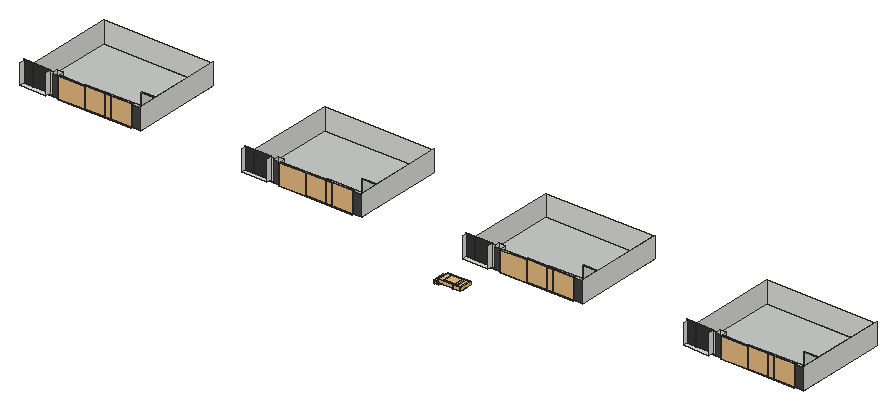
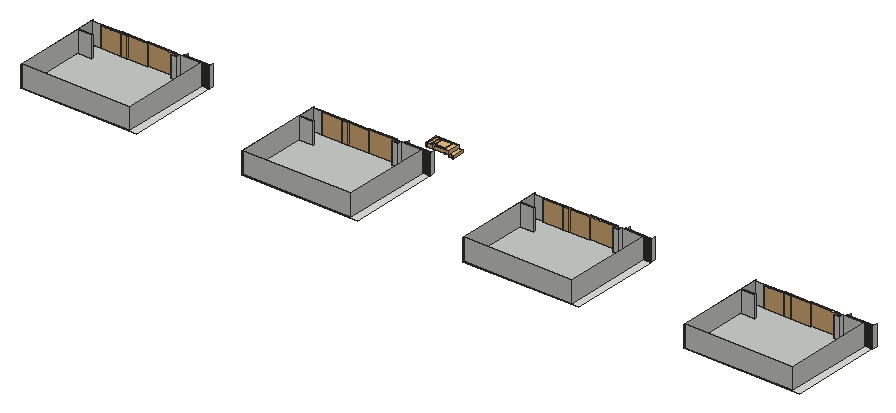
# SketchUp Ruby script. Lengths in inches.
U = 1.inch
M = Sketchup.active_model
def pt(a) = Geom::Point3d.new(a.map { |v| v * U })
def face(e, loops, mat)
  f = e.add_face(loops[0].map { |a| pt(a) })
  loops[1..].each { |l| e.add_face(l.map { |a| pt(a) }).erase! }
  f.material = f.back_material = mat if mat
  f
end
# faces: each face lists its corners as indices into pts; further lists are holes
def faces(e, pts, list, mat = nil) = list.each { |f| face(e, (f[0].is_a?(Array) ? f : [f]).map { |l| l.map { |i| pts[i] } }, mat) }
# xy, xz, yz: faces in a plane at the given z, y or x. An outline is a flat list of corners, or four numbers for a rectangle; further outlines are holes
def ring(l) = l.size == 4 ? [[l[0], l[1]], [l[2], l[1]], [l[2], l[3]], [l[0], l[3]]] : l.each_slice(2).to_a
def flat(e, list, mat, &to3) = list.each { |f| face(e, (f[0].is_a?(Array) ? f : [f]).map { |l| ring(l).map { |u, v| to3.(u, v) } }, mat) }
def xy(e, z, list, mat = nil) = flat(e, list, mat) { |x, y| [x, y, z] }
def xz(e, y, list, mat = nil) = flat(e, list, mat) { |x, z| [x, y, z] }
def yz(e, x, list, mat = nil) = flat(e, list, mat) { |y, z| [x, y, z] }
def lines(e, pts, list) = list.each { |a, b| e.add_line(pt(pts[a]), pt(pts[b])) }
# prism: a flat outline (further loops are holes) pulled along v
def prism(e, loops, v, mat = nil)
  f = face(e, loops, mat); d = Geom::Vector3d.new(v.map { |x| x * U })
  f.pushpull(f.normal.samedirection?(d) ? d.length : -d.length)
end
def box(e, o, s, mat = nil) = prism(e, [[o, [o[0] + s[0], o[1], o[2]], [o[0] + s[0], o[1] + s[1], o[2]], [o[0], o[1] + s[1], o[2]]]], [0, 0, s[2]], mat)
def at(x, y, z, deg = 0) = Geom::Transformation.translation(pt([x, y, z])) * Geom::Transformation.rotation(ORIGIN, Z_AXIS, deg.degrees)
def axes(o, x, y, z) = Geom::Transformation.new([*x, 0, *y, 0, *z, 0, *pt(o).to_a, 1])
def part(name) = M.definitions.add(name)
# library, detail: a bought-in or finely detailed component or shape, given as its bounding box
def library(name, o, s) = part(name).tap { |d| box(d.entities, o, s) }
def detail(e, o, s) = box(e.add_group.entities, o, s)
def put(e, d, t, mat = nil) = e.add_instance(d, t).tap { |i| i.material = mat if mat }
def group(e, t, mat = nil) = e.add_group.tap { |g| g.transformation = t; g.material = mat if mat }.entities
root = M.entities
M.materials.add("[0132_LightGray]").color = [169, 169, 169]
M.materials.add("[0136_Charcoal]2").color = [17, 17, 17]
M.materials.add("[Basic Tile]").color = [203, 206, 202]
M.materials.add("[Granite Dark Gray]").color = [69, 68, 68]
M.materials.add("[Slate Light Tile]").color = [54, 54, 54]
M.materials.add("s600").color = [22, 22, 22]
c1 = library("Group\#649",[0,0,0],[27.27,66.27,16.46])
c2 = library("Group\#647",[0,0,0],[8.93,15.28,7.15])
c3 = library("Scandinavian Door w/ Glass Wall\#2",[-41.94,78.85,0],[6.47,62.99,82.68])
c4 = library("Group\#640",[0,0,0],[35.29,74.27,19.26])
c5 = library("Group\#655",[-5.26,0,0],[129.69,69.79,18.37])
c6 = part("3D_Object__24")
g1 = group(c6.entities,at(-0.5,-39.39,30.52))
p = [[0.5,0,0],[0.5,0.09,0.49],[0.27,0.1875,0.49],[0.15,0.15,0.01],[0.85,0.15,0.01],[0.73,0.1875,0.49],
  [0.18,0.41,0.5],[0,0.5,0.02],[1,0.5,0.02],[0.82,0.41,0.5],[0.27,0.64,0.51],[0.15,0.85,0.04],
  [0.85,0.85,0.04],[0.73,0.64,0.51],[0.5,0.73,0.52],[0.5,1,0.04],[0.5,0.1,0.9],[0.33,0.17,0.9],
  [0.67,0.17,0.9],[0.26,0.34,0.91],[0.74,0.34,0.91],[0.33,0.5,0.91],[0.67,0.5,0.91],[0.5,0.57,0.91],
  [0.34,0.09,1.16],[0.5,0.03,1.16],[0.5,0.24,1.22],[0.66,0.09,1.16],[0.27,0.26,1.17],[0.73,0.26,1.17],
  [0.34,0.42,1.17],[0.5,0.48,1.17],[0.66,0.42,1.17]]
faces(g1,p,[[0,1,2,3],[4,5,1,0],[3,2,6,7],[8,9,5,4],[7,6,10,11],[12,13,9,8],[11,10,14,15],[15,14,13,12],
  [1,16,17,2],[1,5,18,16],[6,2,19],[17,19,2],[9,20,5],[18,5,20],[19,21,6],[20,9,22],
  [10,6,21],[13,22,9],[10,21,14],[23,14,21],[13,14,22],[23,22,14],[24,25,26],[25,27,26],
  [28,24,26],[27,29,26],[30,28,26],[31,30,26],[32,31,26],[29,32,26]])
g2 = group(c6.entities,at(-0.24,-39.37,31.42))
p = [[0.24,0.08,0],[0.24,0,0.26],[0.07,0.07,0.26],[0.07,0.14,0],[0.4,0.14,0],[0.4,0.07,0.26],
  [0.01,0.23,0.27],[0,0.31,0.01],[0.47,0.31,0.01],[0.46,0.23,0.27],[0.07,0.39,0.27],[0.07,0.48,0.01],
  [0.4,0.48,0.01],[0.4,0.39,0.27],[0.24,0.46,0.27],[0.24,0.54,0.01]]
faces(g2,p,[[0,1,2,3],[4,5,1,0],[3,2,6,7],[8,9,5,4],[7,6,10,11],[12,13,9,8],[11,10,14,15],[15,14,13,12]],"[0132_LightGray]")
c7 = library("Group\#660",[0,0,0],[73.87,53.92,3.7])
xy(root,6,[[333.44,581.125,527.2,581.125,527.2,610.99,494.4,610.99,494.4,589.17,376.61,589.17,376.61,1088.45,989.64,1088.45,989.64,690.16,909.32,690.16,909.32,682.59,989.64,682.59,989.64,589.17,939.09,589.17,939.09,581.125,990.19,581.125,990.19,1096.5,333.44,1096.5],[1584.06,581.125,1777.83,581.125,1777.83,610.99,1745.02,610.99,1745.02,589.17,1627.23,589.17,1627.23,1088.45,2240.26,1088.45,2240.26,690.16,2159.95,690.16,2159.95,682.59,2240.26,682.59,2240.26,589.17,2189.71,589.17,2189.71,581.125,2240.81,581.125,2240.81,1096.5,1584.06,1096.5],[2834.69,581.125,3028.45,581.125,3028.45,610.99,2995.65,610.99,2995.65,589.17,2877.86,589.17,2877.86,1088.45,3490.89,1088.45,3490.89,690.16,3410.57,690.16,3410.57,682.59,3490.89,682.59,3490.89,589.17,3440.34,589.17,3440.34,581.125,3491.44,581.125,3491.44,1096.5,2834.69,1096.5],[4085.31,581.125,4279.08,581.125,4279.08,610.99,4246.27,610.99,4246.27,589.17,4128.48,589.17,4128.48,1088.45,4741.51,1088.45,4741.51,690.16,4661.2,690.16,4661.2,682.59,4741.51,682.59,4741.51,589.17,4690.96,589.17,4690.96,581.125,4742.06,581.125,4742.06,1096.5,4085.31,1096.5]])
xy(root,6,[[527.2,580.3125,939.09,580.3125,939.09,589.17,989.64,589.17,989.64,682.59,909.32,682.59,909.32,690.16,989.64,690.16,989.64,1088.45,376.61,1088.45,376.61,589.17,494.4,589.17,494.4,610.99,527.2,610.99],[1777.83,580.3125,2189.71,580.3125,2189.71,589.17,2240.26,589.17,2240.26,682.59,2159.95,682.59,2159.95,690.16,2240.26,690.16,2240.26,1088.45,1627.23,1088.45,1627.23,589.17,1745.02,589.17,1745.02,610.99,1777.83,610.99],[3028.45,580.3125,3440.34,580.3125,3440.34,589.17,3490.89,589.17,3490.89,682.59,3410.57,682.59,3410.57,690.16,3490.89,690.16,3490.89,1088.45,2877.86,1088.45,2877.86,589.17,2995.65,589.17,2995.65,610.99,3028.45,610.99],[4279.08,580.3125,4690.96,580.3125,4690.96,589.17,4741.51,589.17,4741.51,682.59,4661.2,682.59,4661.2,690.16,4741.51,690.16,4741.51,1088.45,4128.48,1088.45,4128.48,589.17,4246.27,589.17,4246.27,610.99,4279.08,610.99]],"[Basic Tile]")
xy(root,11.5,[[327.6,559.875,474.41,586.25],[1578.23,559.875,1725.04,586.25],[2828.85,559.875,2975.66,586.25],[4079.48,559.875,4226.29,586.25]])
xz(root,580.3125,[[527.2,1.19,939.09,6],[1777.83,1.19,2189.71,6],[3028.45,1.19,3440.34,6],[4279.08,1.19,4690.96,6]],"[Granite Dark Gray]")
xz(root,581.125,[[492.21,6,527.2,120.25],[939.09,6,990.19,120.25],[1742.84,6,1777.83,120.25],[2189.71,6,2240.81,120.25],[2993.46,6,3028.45,120.25],
  [3440.34,6,3491.44,120.25],[4244.09,6,4279.08,120.25],[4690.96,6,4742.06,120.25]],"[Granite Dark Gray]")
xz(root,586.25,[[327.6,11.5,474.41,132],[1578.23,11.5,1725.04,132],[2828.85,11.5,2975.66,132],[4079.48,11.5,4226.29,132]],"[Slate Light Tile]")
xz(root,589.17,[[376.61,6,494.4,126],[939.09,6,939.09,120.25,810.34,120.25,810.34,126,989.64,126,989.64,6],[1627.23,6,1745.02,126],[2189.71,6,2189.71,120.25,2060.96,120.25,2060.96,126,2240.26,126,2240.26,6],[2877.86,6,2995.65,126],
  [3440.34,6,3440.34,120.25,3311.59,120.25,3311.59,126,3490.89,126,3490.89,6],[4128.48,6,4246.27,126],[4690.96,6,4690.96,120.25,4562.21,120.25,4562.21,126,4741.51,126,4741.51,6]])
xz(root,610.99,[[494.4,6,527.2,126],[1745.02,6,1777.83,126],[2995.65,6,3028.45,126],[4246.27,6,4279.08,126]])
xz(root,682.59,[[909.32,6,989.64,126],[2159.95,6,2240.26,126],[3410.57,6,3490.89,126],[4661.2,6,4741.51,126]],"[Basic Tile]")
xz(root,690.16,[[909.32,6,989.64,126],[2159.95,6,2240.26,126],[3410.57,6,3490.89,126],[4661.2,6,4741.51,126]])
xz(root,1088.45,[[376.61,6,989.64,126],[1627.23,6,2240.26,126],[2877.86,6,3490.89,126],[4128.48,6,4741.51,126]])
yz(root,327.6,[[559.875,11.5,586.25,126]])
yz(root,376.61,[[589.17,6,1088.45,126]])
yz(root,474.41,[[559.875,11.5,586.25,126]])
yz(root,494.4,[[589.17,6,610.99,126]])
yz(root,527.2,[[580.3125,1.19,581.125,6],[581.125,6,610.99,120.25]])
yz(root,909.32,[[682.59,6,690.16,126]],"[Basic Tile]")
yz(root,939.09,[[580.3125,1.19,581.125,6],[581.125,6,589.17,120.25]])
yz(root,989.64,[[690.16,6,1088.45,126]])
yz(root,989.64,[[589.17,6,682.59,126]],"[Basic Tile]")
yz(root,990.19,[[581.125,6,1096.5,126]])
yz(root,1578.23,[[559.875,11.5,586.25,126]])
yz(root,1627.23,[[589.17,6,1088.45,126]])
yz(root,1725.04,[[559.875,11.5,586.25,126]])
yz(root,1745.02,[[589.17,6,610.99,126]])
yz(root,1777.83,[[580.3125,1.19,581.125,6],[581.125,6,610.99,120.25]])
yz(root,2159.95,[[682.59,6,690.16,126]],"[Basic Tile]")
yz(root,2189.71,[[580.3125,1.19,581.125,6],[581.125,6,589.17,120.25]])
yz(root,2240.26,[[690.16,6,1088.45,126]])
yz(root,2240.26,[[589.17,6,682.59,126]],"[Basic Tile]")
yz(root,2240.81,[[581.125,6,1096.5,126]])
yz(root,2828.85,[[559.875,11.5,586.25,126]])
yz(root,2877.86,[[589.17,6,1088.45,126]])
yz(root,2975.66,[[559.875,11.5,586.25,126]])
yz(root,2995.65,[[589.17,6,610.99,126]])
yz(root,3028.45,[[580.3125,1.19,581.125,6],[581.125,6,610.99,120.25]])
yz(root,3410.57,[[682.59,6,690.16,126]],"[Basic Tile]")
yz(root,3440.34,[[580.3125,1.19,581.125,6],[581.125,6,589.17,120.25]])
yz(root,3490.89,[[690.16,6,1088.45,126]])
yz(root,3490.89,[[589.17,6,682.59,126]],"[Basic Tile]")
yz(root,3491.44,[[581.125,6,1096.5,126]])
yz(root,4079.48,[[559.875,11.5,586.25,126]])
yz(root,4128.48,[[589.17,6,1088.45,126]])
yz(root,4226.29,[[559.875,11.5,586.25,126]])
yz(root,4246.27,[[589.17,6,610.99,126]])
yz(root,4279.08,[[580.3125,1.19,581.125,6],[581.125,6,610.99,120.25]])
yz(root,4661.2,[[682.59,6,690.16,126]],"[Basic Tile]")
yz(root,4690.96,[[580.3125,1.19,581.125,6],[581.125,6,589.17,120.25]])
yz(root,4741.51,[[690.16,6,1088.45,126]])
yz(root,4741.51,[[589.17,6,682.59,126]],"[Basic Tile]")
yz(root,4742.06,[[581.125,6,1096.5,126]])
put(root,c1,at(2883.05,390.43,1.17,-179.359))
put(root,c2,at(2864.7,393.04,1.88,-179.359),"s600")
put(root,c2,axes([2865.51,321.15,1.88],[-0.99994,-0.01119,0],[-0.01119,0.99994,0],[0,0,1]),"s600")
put(root,c3,axes([3288.94,516.22,265.5625],[0,-1.83,0],[0,0,-1.83],[1.83,0,0]),"[Basic Tile]")
put(root,c3,axes([4539.57,516.22,265.5625],[0,-1.83,0],[0,0,-1.83],[1.83,0,0]),"[Basic Tile]")
put(root,c3,axes([787.69,516.22,265.5625],[0,-1.83,0],[0,0,-1.83],[1.83,0,0]),"[Basic Tile]")
put(root,c3,axes([2038.32,516.22,265.5625],[0,-1.83,0],[0,0,-1.83],[1.83,0,0]),"[Basic Tile]")
put(root,c3,axes([3028.45,510.84,265.5625],[0,-1.83,0],[0,0,-1.83],[1.83,0,0]))
put(root,c3,axes([3174.89,515.49,265.5625],[0,-1.83,0],[0,0,-1.83],[1.83,0,0]),"[Basic Tile]")
put(root,c3,axes([4279.08,510.84,265.5625],[0,-1.83,0],[0,0,-1.83],[1.83,0,0]))
put(root,c3,axes([4425.51,515.49,265.5625],[0,-1.83,0],[0,0,-1.83],[1.83,0,0]),"[Basic Tile]")
put(root,c3,axes([527.2,510.84,265.5625],[0,-1.83,0],[0,0,-1.83],[1.83,0,0]))
put(root,c3,axes([673.64,515.49,265.5625],[0,-1.83,0],[0,0,-1.83],[1.83,0,0]),"[Basic Tile]")
put(root,c3,axes([1924.26,515.49,265.5625],[0,-1.83,0],[0,0,-1.83],[1.83,0,0]),"[Basic Tile]")
put(root,c3,axes([1777.83,510.84,265.5625],[0,-1.83,0],[0,0,-1.83],[1.83,0,0]))
put(root,c4,at(3002.9,395.77,12.92,-179.359))
put(root,c5,at(3004.37,393.55,12.98,-179.359),"s600")
g3 = group(root,at(3010.3,393.7,12.98,-179.359),"s600")
p = [[6.73,0,0.1],[6.125,2.06,0.02],[5.51,2.32,0.36],[7.04,0.08,0],[4.43,4.6,0.63],[5.38,4.27,0.11],
  [4.43,65.35,0.63],[6.125,67.89,0.02],[5.51,67.63,0.36],[5.38,65.68,0.11],[6.73,69.95,0.1],[7.04,69.87,0],
  [3.54,11.56,0.11],[2.8125,11.41,1.02],[1.48,18.64,1.39],[2.14,18.85,0.5],[3.54,58.39,0.11],[1.48,51.3125,1.39],
  [2.14,51.1,0.5],[2.8125,58.54,1.02],[1.16,26.91,0.5],[0.49,26.81,1.67],[0,34.98,1.75],[0.68,34.98,0.5],
  [1.16,43.04,0.5],[0.49,43.14,1.67]]
faces(g3,p,[[0,1,2],[1,0,3],[1,4,2],[4,1,5],[6,7,8],[7,6,9],[7,10,8],[10,7,11],
  [12,4,5],[4,12,13],[12,14,13],[14,12,15],[16,17,18],[17,16,19],[16,6,19],[6,16,9],
  [14,20,21],[20,14,15],[20,22,21],[22,20,23],[24,22,23],[22,24,25],[24,17,25],[17,24,18]],"[0136_Charcoal]2")
g4 = group(root,at(2899.79,320.26,13.35))
yz(g4,3.61,[[0.6875,0.72,0.2,1.02,0.28,1.23,0.77,0.92]],"[0132_LightGray]")
p = [[3.5,0.38,-0.04],[4.45,0.35,-0.05],[4.45,-0.14,0.25],[3.49,-0.11,0.26],[4.61,0.4375,0.17],[4.61,-0.05,0.47],
  [3.5,0.39,-0.03],[4.03,0.55,0.4],[4.11,0.58,0.49],[4.14,0.62,0.58],[4.12,0.64,0.65],[4.05,0.67,0.7],
  [3.95,0.68,0.73],[3.82,0.69,0.74],[3.73,0.69,0.74],[3.61,0.6875,0.72],[3.61,0.77,0.92],[3.77,0.77,0.94],
  [3.92,0.77,0.95],[4.04,0.76,0.94],[4.16,0.75,0.92],[4.26,0.74,0.89],[4.35,0.72,0.85],[4.42,0.7,0.81],
  [4.47,0.68,0.75],[4.5,0.65,0.69],[4.51,0.625,0.625],[4.47,0.57,0.5],[4.375,0.53,0.38],[4.15,0.45,0.17],
  [2.63,0.65,0.56],[2.62,0.41,-0.04],[2.62,-0.08,0.27],[2.63,0.16,0.86],[2.95,0.4,-0.04],[2.95,-0.09,0.26],
  [2.97,0.79,0.93],[2.96,0.3,1.23],[3.49,-0.1,0.27],[4.02,0.06,0.71],[0.05,0.9,0.98],[0.95,0.47,-0.02],
  [0.95,-0.02,0.28],[0.04,0.41,1.28],[1.4,0.45,-0.03],[1.39,-0.04,0.27],[2.35,0.82,0.96],[2.34,0.33,1.26],
  [2.51,0.64,0.51],[2.375,0.63,0.48],[2.38,0.72,0.7],[2.48,0.73,0.75],[2.57,0.75,0.8],[2.65,0.77,0.86],
  [2.7,0.8,0.93],[0.67,0.88,0.97],[1.1875,0.62,0.36],[1.73,0.84,0.96],[4.14,-0.04,0.48],[4.37,0.04,0.68],
  [2.7,0.31,1.23],[2.64,0.28,1.16],[2.57,0.26,1.1],[2.48,0.24,1.05],[2.375,0.23,1],[2.37,0.14,0.78],
  [2.5,0.15,0.8125],[4.47,0.08,0.8],[4.5,0.13,0.93],[4.49,0.16,0.99],[4.46,0.18,1.05],[4.41,0.21,1.11],
  [4.34,0.23,1.16],[4.25,0.25,1.2],[4.15,0.26,1.22],[4.04,0.27,1.24],[3.91,0.28,1.25],[3.76,0.28,1.24],
  [3.61,0.28,1.23],[3.61,0.2,1.02],[3.72,0.2,1.04],[3.82,0.2,1.05],[3.95,0.19,1.03],[4.04,0.18,1],
  [4.11,0.15,0.95],[4.14,0.125,0.88],[4.11,0.09,0.8],[1.72,0.35,1.27],[1.18,0.125,0.67],[0.66,0.39,1.27]]
faces(g4,p,[[0,1,2,3],[1,4,5,2],[4,1,0,6,7,8,9,10,11,12,13,14,15,16,17,18,19,20,21,22,23,24,25,26,27,28,29],[30,31,32,33],[31,34,35,32],[34,36,37,35],[7,6,38,39],[6,0,3,38],
  [40,41,42,43],[41,44,45,42],[44,46,47,45],[34,31,30,48,49,50,51,52,53,54,36],[46,44,41,40,55,56,57],[4,29,58,5],[29,28,59,58],[32,35,37,60,61,62,63,64,65,66,33],
  [2,5,58,59,67,68,69,70,71,72,73,74,75,76,77,78,79,80,81,82,83,84,85,86,39,38,3],[45,47,87,88,89,43,42],[28,27,67,59],[56,55,89,88],[57,56,88,87],[8,7,39,86],[50,49,65,64],[49,48,66,65],
  [48,30,33,66],[9,8,86,85],[27,26,68,67],[10,9,85,84],[26,25,69,68],[11,10,84,83],[51,50,64,63],[52,51,63,62],
  [15,14,80,79],[14,13,81,80],[13,12,82,81],[12,11,83,82],[25,24,70,69],[23,22,72,71],[24,23,71,70],[53,52,62,61],
  [21,20,74,73],[22,21,73,72],[54,53,61,60],[36,54,60,37],[17,16,78,77],[18,17,77,76],[19,18,76,75],[20,19,75,74],
  [46,57,87,47],[55,40,43,89]],"[0132_LightGray]")
g5 = group(root,at(2901.78,394.76,13.27,-179.359))
prism(g5,[[[2.93,0.74,0.01],[2.6,0.73,0.02],[2.59,0.95,0.63],[2.47,0.93,0.59],[2.34,0.91,0.55],[2.34,1,0.78],[2.44,1.02,0.83],[2.53,1.04,0.88],[2.6,1.07,0.95],[2.65,1.1,1.02],[2.92,1.1,1.01]]],[0.02,-0.67,0.25],"[0132_LightGray]")
prism(g5,[[[4.58,0.875,0.23],[4.43,0.79,0],[3.47,0.76,0.01],[3.47,0.76,0.02],[3.99,0.94,0.47],[4.07,0.98,0.57],[4.1,1.01,0.65],[4.08,1.04,0.73],[4.01,1.06,0.78],[3.91,1.07,0.8125],[3.78,1.07,0.83],[3.68,1.06,0.82],[3.57,1.05,0.8],[3.57,1.13,1.01],[3.72,1.14,1.03],[3.87,1.15,1.04],[4,1.15,1.03],[4.11,1.15,1.01],[4.21,1.14,0.98],[4.3,1.125,0.94],[4.37,1.11,0.89],[4.42,1.09,0.83],[4.45,1.07,0.77],[4.47,1.05,0.7],[4.43,1,0.57],[4.34,0.95,0.45],[4.12,0.86,0.23]]],[0.02,-0.67,0.25],"[0132_LightGray]")
prism(g5,[[[2.3,1.1,1.05],[1.37,0.6875,0.03],[0.93,0.67,0.03],[0,1.02,1.07],[0.62,1.04,1.0625],[1.15,0.83,0.43],[1.68,1.08,1.05]]],[0.02,-0.67,0.25],"[0132_LightGray]")
g6 = group(root,at(2857.9375,388.78,13.9375,-179.359),"s600")
prism(g6,[[[0.58,63.0625,0.1],[0.55,62.99,0.11],[0.51,62.93,0.13],[0.45,62.89,0.14],[0.375,62.86,0.15],[0.3,62.85,0.15],[0.22,62.86,0.15],[0.15,62.88,0.14],[0.09,62.93,0.13],[0.04,62.99,0.12],[0.01,63.06,0.1],[0,63.13,0.08],[0.01,63.2,0.06],[0.04,63.27,0.04],[0.08,63.33,0.02],[0.14,63.38,0.01],[0.22,63.41,0],[0.29,63.42,0],[0.37,63.41,0],[0.44,63.38,0.01],[0.5,63.34,0.02],[0.55,63.28,0.04],[0.58,63.21,0.06],[0.59,63.14,0.08]]],[0,0.1,0.38],"[0132_LightGray]")
prism(g6,[[[0.55,0.53,0.11],[0.58,0.46,0.1],[0.59,0.38,0.08],[0.58,0.31,0.06],[0.55,0.24,0.04],[0.5,0.18,0.02],[0.44,0.14,0.01],[0.37,0.11,0],[0.29,0.1,0],[0.22,0.11,0],[0.14,0.14,0.01],[0.08,0.1875,0.02],[0.04,0.25,0.04],[0.01,0.32,0.06],[0,0.39,0.08],[0.01,0.46,0.1],[0.04,0.53,0.12],[0.09,0.59,0.13],[0.15,0.64,0.14],[0.22,0.66,0.15],[0.3,0.67,0.15],[0.375,0.66,0.15],[0.45,0.63,0.14],[0.51,0.59,0.13]]],[0,-0.1,0.38],"[0132_LightGray]")
put(root,c6,axes([2880.88,341.56,-38.91],[-1.28992,-0.01444,0],[0.01444,-1.28992,0],[0,0,1.77735]),"s600")
g7 = group(root,at(2883.42,357.3,16.55,-179.359),"s600")
p = [[1.77,27.6,0.3125],[0.24,32.57,0.13],[0,32.46,0],[2.08,27.64,0.49],[2.87,20.64,0.73],[2.55,20.64,0.58],
  [3.26,11.29,0.94],[3,11.29,0.84],[3.39,0,1.09],[3.08,0,0.92]]
faces(g7,p,[[0,1,2],[1,0,3],[0,4,3],[4,0,5],[6,5,7],[5,6,4],[7,8,6],[8,7,9]])
g8 = group(root,at(2910.81,390.74,16.55,-179.359))
p = [[28,0.57,0.13],[27.76,0.67,0],[19.65,2.125,4.48],[27.76,65.59,0],[28,65.7,0.13],[19.65,64.14,4.48],
  [19.86,2.01,4.34],[27.79,0,0.09],[20.18,1.33,4],[19.86,64.25,4.34],[20.18,64.93,4],[27.79,66.27,0.09],
  [14.65,2.55,6.89],[14.65,63.72,6.89],[14.53,3.2,7.125],[14.53,63.0625,7.125],[14.29,3.3,7.125],[14.29,62.96,7.125],
  [8.96,4.58,10.03],[9.12,3.9,9.78],[8.96,61.6875,10.03],[9.12,62.37,9.78],[8.75,4.68,10.03],[8.75,61.59,10.03],
  [4.71,5.02,11.96],[4.71,61.25,11.96],[4.8,5.69,12.05],[4.59,5.81,12.05],[4.8,60.57,12.05],[4.59,60.46,12.05],
  [0,6.3,14.13],[0.33,6.78,14],[0.44,6.82,13.9375],[0.44,59.45,13.9375],[0.33,59.49,14],[0,59.97,14.13]]
faces(g8,p,[[0,1,2],[3,4,5],[0,6,7],[6,8,7],[0,2,6],[5,4,9],[10,9,11],[9,4,11],
  [6,12,8],[13,9,10],[12,6,14],[2,14,6],[9,13,15],[15,5,9],[14,2,16],[5,15,17],
  [18,12,14],[12,18,19],[13,20,15],[20,13,21],[16,18,14],[18,16,22],[17,20,23],[20,17,15],
  [18,24,19],[25,20,21],[24,18,26],[22,26,18],[26,22,27],[23,28,29],[20,25,28],[28,23,20],
  [26,30,24],[30,26,31],[27,31,26],[27,32,31],[33,29,34],[28,35,34],[34,29,28],[35,28,25]],"[0136_Charcoal]2")
g9 = group(root,at(2883.05,389.86,16.55,-179.359),"s600")
p = [[0.24,0,0.13],[1.77,4.96,0.3125],[0,0.11,0],[2.08,4.93,0.49],[2.87,11.92,0.73],[2.55,11.92,0.58],
  [3.26,21.27,0.94],[3,21.27,0.84],[3.39,32.57,1.09],[3.08,32.57,0.92]]
faces(g9,p,[[0,1,2],[1,0,3],[4,1,3],[1,4,5],[6,5,4],[5,6,7],[8,7,6],[7,8,9]])
put(root,c7,at(2982.84,385.375,29.91,-179.359))
